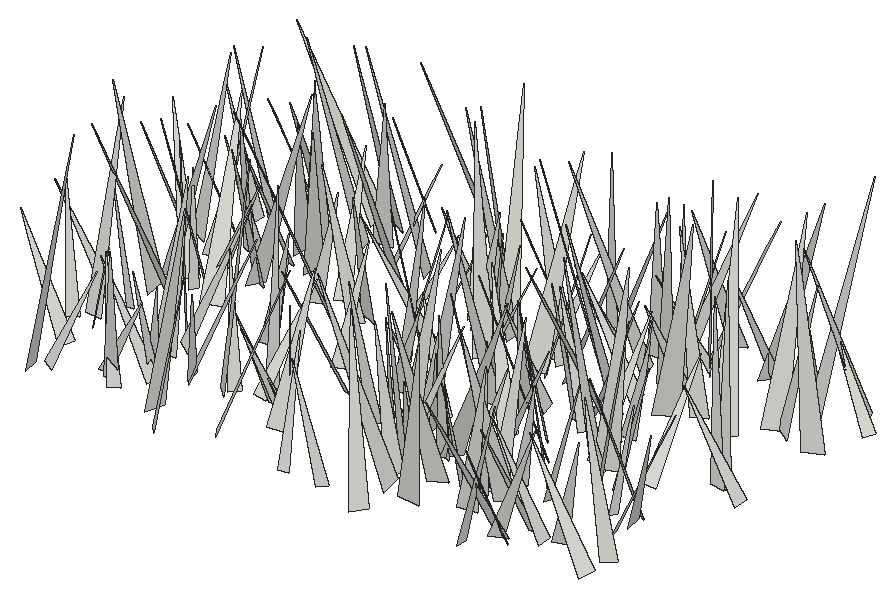
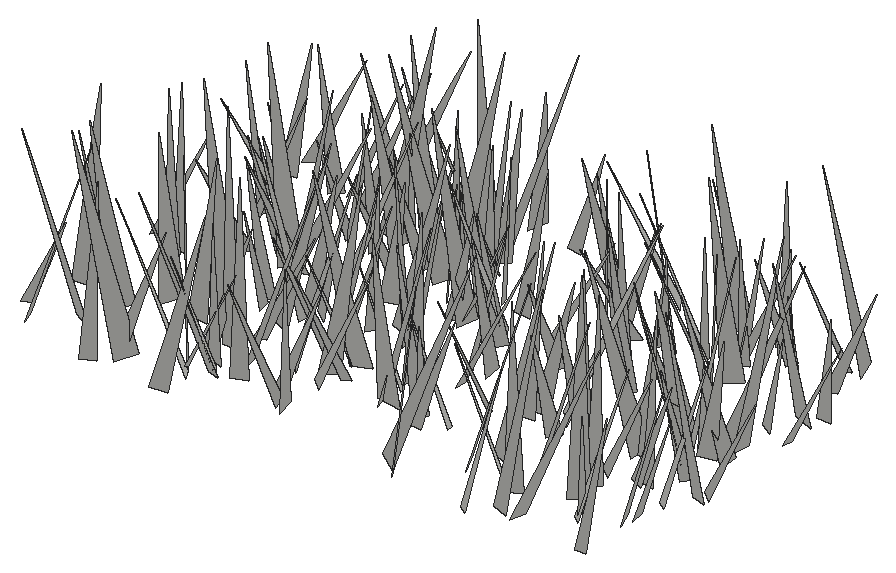
# SketchUp Ruby script. Lengths in inches.
U = 1.inch
M = Sketchup.active_model
def pt(a) = Geom::Point3d.new(a.map { |v| v * U })
def face(e, loops, mat)
  f = e.add_face(loops[0].map { |a| pt(a) })
  loops[1..].each { |l| e.add_face(l.map { |a| pt(a) }).erase! }
  f.material = f.back_material = mat if mat
  f
end
# faces: each face lists its corners as indices into pts; further lists are holes
def faces(e, pts, list, mat = nil) = list.each { |f| face(e, (f[0].is_a?(Array) ? f : [f]).map { |l| l.map { |i| pts[i] } }, mat) }
# xy, xz, yz: faces in a plane at the given z, y or x. An outline is a flat list of corners, or four numbers for a rectangle; further outlines are holes
def ring(l) = l.size == 4 ? [[l[0], l[1]], [l[2], l[1]], [l[2], l[3]], [l[0], l[3]]] : l.each_slice(2).to_a
def flat(e, list, mat, &to3) = list.each { |f| face(e, (f[0].is_a?(Array) ? f : [f]).map { |l| ring(l).map { |u, v| to3.(u, v) } }, mat) }
def xy(e, z, list, mat = nil) = flat(e, list, mat) { |x, y| [x, y, z] }
def xz(e, y, list, mat = nil) = flat(e, list, mat) { |x, z| [x, y, z] }
def yz(e, x, list, mat = nil) = flat(e, list, mat) { |y, z| [x, y, z] }
def lines(e, pts, list) = list.each { |a, b| e.add_line(pt(pts[a]), pt(pts[b])) }
# prism: a flat outline (further loops are holes) pulled along v
def prism(e, loops, v, mat = nil)
  f = face(e, loops, mat); d = Geom::Vector3d.new(v.map { |x| x * U })
  f.pushpull(f.normal.samedirection?(d) ? d.length : -d.length)
end
def box(e, o, s, mat = nil) = prism(e, [[o, [o[0] + s[0], o[1], o[2]], [o[0] + s[0], o[1] + s[1], o[2]], [o[0], o[1] + s[1], o[2]]]], [0, 0, s[2]], mat)
def at(x, y, z, deg = 0) = Geom::Transformation.translation(pt([x, y, z])) * Geom::Transformation.rotation(ORIGIN, Z_AXIS, deg.degrees)
def axes(o, x, y, z) = Geom::Transformation.new([*x, 0, *y, 0, *z, 0, *pt(o).to_a, 1])
def part(name) = M.definitions.add(name)
# library, detail: a bought-in or finely detailed component or shape, given as its bounding box
def library(name, o, s) = part(name).tap { |d| box(d.entities, o, s) }
def detail(e, o, s) = box(e.add_group.entities, o, s)
def put(e, d, t, mat = nil) = e.add_instance(d, t).tap { |i| i.material = mat if mat }
def group(e, t, mat = nil) = e.add_group.tap { |g| g.transformation = t; g.material = mat if mat }.entities
root = M.entities
c1 = part("fur_instance\#9")
p = [[0.8125,0,1.79],[0.67,-0.02,1.48],[0,-0.11,0],[0,0.11,0]]
faces(c1.entities,p,[[0,1,2,3]])
put(root,c1,axes([494.67,199.78,-21.66],[-2.5051,-3.46967,0.23869],[-3.39401,2.50314,0.76559],[0.75915,-0.25846,4.21047]))
put(root,c1,axes([494.2,200.04,-21.66],[-1.56968,-5.60909,0.11931],[-5.50885,1.51747,-1.1357],[-1.06238,0.41882,5.71278]))
put(root,c1,axes([481.14,198.01,-21.66],[-1.35537,3.98703,1.26023],[4.07237,0.95801,1.34893],[-0.94888,-1.58348,3.98921]))
put(root,c1,axes([468.15,197.01,-21.66],[3.87453,3.49507,1.24049],[3.40824,-4.0629,0.80191],[-1.46226,-0.20898,5.15601]))
put(root,c1,axes([484.87,197.01,-21.66],[-6.05277,2.56522,0.71834],[2.46544,6.06973,-0.90131],[1.00895,0.55714,6.51184]))
put(root,c1,axes([492.67,197.71,-21.66],[4.75143,0.92242,1.33841],[0.70934,-4.89704,0.85681],[-1.46255,0.62163,4.7637]))
put(root,c1,axes([486.59,199.97,-21.66],[1.17018,-6.95871,1.51726],[-7.0392,-0.89595,1.31981],[1.08411,1.69372,6.93189]))
put(root,c1,axes([462.06,200.32,-21.66],[-0.22733,-5.68785,1.31588],[-5.73337,0.46581,1.02292],[1.10075,1.2515,5.59972]))
put(root,c1,axes([501.49,199.53,-21.66],[-4.58774,2.19144,0.09862],[2.15217,4.45217,1.18567],[-0.42461,-1.11142,4.94408]))
put(root,c1,axes([477.98,197.96,-21.66],[0.35019,4.61175,0.40741],[4.56098,-0.41379,0.76359],[-0.79477,-0.34263,4.56155]))
put(root,c1,axes([493.86,199.77,-21.66],[3.98681,-3.04122,0.56389],[-3.08769,-3.85909,1.01744],[0.18196,1.14894,4.91004]))
put(root,c1,axes([484.51,200.73,-21.66],[-7.8071,-1.03462,1.04066],[-0.93299,7.84786,0.80297],[1.13267,-0.66693,7.83431]))
put(root,c1,axes([466.49,199.24,-21.66],[7.07212,-1.1156,2.41076],[-1.38462,-7.39913,0.63784],[-2.26697,1.03896,7.1311]))
put(root,c1,axes([457.67,199.39,-21.66],[1.33461,3.80482,0.72121],[3.71713,-1.04467,-1.36733],[1.08616,-1.09999,3.79319]))
put(root,c1,axes([456.9,198.5625,-21.66],[7.33246,2.99097,2.42144],[2.72494,-7.71469,1.27771],[-2.71735,0.33456,7.81527]))
put(root,c1,axes([496.68,201.2,-21.66],[-4.54566,0.43172,0.55069],[0.54174,4.46219,0.97364],[0.44289,-1.02717,4.4611]))
put(root,c1,axes([495.29,201.81,-21.66],[-1.01525,-4.25558,0.24661],[-4.20456,0.95799,-0.77812],[-0.70176,0.41691,4.30525]))
put(root,c1,axes([462.74,199.7,-21.66],[-1.18349,4.29439,0.91251],[4.36217,1.04349,0.74676],[-0.49586,-1.06979,4.39144]))
put(root,c1,axes([490.27,201.32,-21.66],[2.54415,-5.74451,1.38415],[-5.89364,-2.3587,1.04378],[0.42454,1.68081,6.19537]))
put(root,c1,axes([461.02,200.97,-21.66],[2.09245,-2.98815,0.44058],[-2.87886,-1.81085,1.39087],[0.91397,1.13723,3.37237]))
put(root,c1,axes([497.64,201.65,-21.66],[2.67886,-4.09104,0.57639],[-4.11516,-2.58128,0.80469],[0.36641,0.91951,4.82342]))
put(root,c1,axes([471.55,199.15,-21.66],[5.03516,3.5658,0.22039],[3.50469,-5.00395,0.89105],[-0.69327,0.6016,6.10523]))
put(root,c1,axes([486.55,203.04,-21.66],[1.44091,-6.85532,1.40735],[-6.89305,-1.6385,-0.92385],[-1.20912,1.1714,6.94393]))
put(root,c1,axes([464.1,202.01,-21.66],[-4.45422,0.97791,0.2811],[1.01486,4.3608,0.91044],[0.07343,-0.95002,4.4685]))
put(root,c1,axes([483.74,202.0625,-21.66],[3.52477,-3.78027,2.43443],[-3.94318,-4.08529,-0.63451],[-2.1606,1.28874,5.1295]))
put(root,c1,axes([463.72,202.64,-21.66],[-3.9744,-0.24759,1.6573],[0.13335,4.20562,0.94807],[1.67038,-0.92483,3.8676]))
put(root,c1,axes([491.44,203.78,-21.66],[2.47706,-6.70826,1.39737],[-6.69174,-2.68793,-1.04158],[-1.47445,0.92925,7.07472]))
put(root,c1,axes([463.31,203.02,-21.66],[0.57309,-4.07864,0.58369],[-4.03575,-0.43699,0.90892],[0.82985,0.69149,4.01716]))
put(root,c1,axes([501.54,201.7,-21.66],[-2.10663,5.00928,1.58804],[5.23429,1.84857,1.1125],[-0.46582,-1.88217,5.31913]))
put(root,c1,axes([456.88,202.27,-21.66],[-3.88022,2.75048,0.41463],[2.75578,3.70465,1.21426],[-0.37781,-1.22622,4.59857]))
put(root,c1,axes([483.27,204.12,-21.66],[4.01305,-1.4697,0.35123],[-1.33059,-3.90931,-1.15533],[-0.71618,-0.97223,4.11458]))
put(root,c1,axes([484.54,202.18,-21.66],[-3.5063,-5.04513,2.56803],[-5.65565,3.25438,-1.32851],[0.24851,2.88062,5.99854]))
put(root,c1,axes([474.17,203.42,-21.66],[-3.42009,-2.62307,1.97794],[-2.56254,3.91671,0.76324],[2.05575,0.51835,4.24205]))
put(root,c1,axes([465.8,203.89,-21.66],[3.91592,-0.46866,0.80636],[-0.26131,-3.89224,-0.99321],[-0.89531,-0.91384,3.81675]))
put(root,c1,axes([474.28,201.85,-21.66],[-2.07384,5.25709,1.74566],[5.26815,2.4479,-1.11335],[1.712,-1.16445,5.54061]))
put(root,c1,axes([488.96,202.72,-21.66],[0.98464,3.25356,1.70885],[3.23357,-1.6077,1.19779],[-1.74639,-1.14237,3.18127]))
put(root,c1,axes([472.22,204.58,-21.66],[-3.37943,-0.96857,0.84627],[-0.6019,3.29348,1.36586],[1.13667,-1.13567,3.23931]))
put(root,c1,axes([471.98,204.55,-21.66],[0.37183,-3.94608,0.38846],[-3.8933,-0.43727,-0.71534],[-0.75144,0.31297,3.89847]))
put(root,c1,axes([483.19,203.37,-21.66],[2.79379,4.96818,0.70977],[4.95175,-2.59669,-1.31495],[0.8165,-1.25148,5.54607]))
put(root,c1,axes([465.8,203.64,-21.66],[4.98455,3.49636,0.32674],[3.50629,-4.92427,-0.79656],[0.19289,-0.83908,6.03621]))
put(root,c1,axes([456.49,205.47,-21.66],[3.46775,1.51161,0.84573],[1.722,-3.21287,-1.3182],[-0.18693,-1.55498,3.54578]))
put(root,c1,axes([489.76,203.69,-21.66],[1.9045,4.44389,1.45881],[4.34306,-2.26488,1.22946],[-1.73613,-0.79091,4.67587]))
put(root,c1,axes([462.55,205.04,-21.66],[2.84119,-6.18581,2.36185],[-6.62137,-2.65127,1.02137],[0.00779,2.57322,6.73004]))
put(root,c1,axes([484.66,205.87,-21.66],[-1.17903,-5.46423,1.73554],[-5.62366,1.44698,0.7353],[1.11548,1.51937,5.54141]))
put(root,c1,axes([468.48,203.64,-21.66],[5.2038,5.70361,2.35891],[5.67233,-5.63566,1.11317],[-2.43315,-0.93989,7.64013]))
put(root,c1,axes([480.47,206.04,-21.66],[4.23333,1.58778,2.03705],[2.11026,-4.38143,-0.97034],[-1.48911,-1.69519,4.41595]))
put(root,c1,axes([499.62,206.57,-21.66],[4.97063,-0.22915,0.23226],[-0.15729,-4.7897,-1.3593],[-0.28585,-1.34904,4.78665]))
put(root,c1,axes([490.78,206.12,-21.66],[2.11868,-4.0714,0.72457],[-4.11944,-2.00647,0.77101],[0.3627,0.99394,4.52445]))
put(root,c1,axes([469.07,204.14,-21.66],[-4.35702,1.54483,0.37411],[1.45493,4.3157,-0.87633],[0.64002,0.7059,4.53896]))
put(root,c1,axes([485.13,206.16,-21.66],[6.73019,-3.63445,0.24466],[-3.63894,-6.68481,0.79754],[0.16506,0.81773,7.60715]))
put(root,c1,axes([490.28,204.5,-21.66],[-4.55508,3.55475,2.05706],[3.40532,4.98624,-1.07596],[2.29598,-0.34303,5.67691]))
put(root,c1,axes([478.51,206.57,-21.66],[-0.10037,-5.00985,1.67679],[-5.24561,-0.10471,-0.62683],[-0.62754,1.67652,4.9715]))
put(root,c1,axes([493.1,206.13,-21.66],[-3.89447,-3.70378,1.65585],[-4.00703,3.87088,-0.766],[0.63525,1.71028,5.3196]))
put(root,c1,axes([454.92,205.32,-21.66],[-0.91318,4.58049,0.90258],[4.61205,0.74242,0.89849],[-0.72428,-1.04754,4.5834]))
put(root,c1,axes([487.09,205.95,-21.66],[3.48145,-1.92251,0.90917],[-2.10367,-3.36896,0.93158],[-0.31179,1.26381,3.86636]))
put(root,c1,axes([499.5,204.74,-21.66],[4.18382,1.92252,0.07247],[1.86113,-4.08842,1.01327],[-0.48737,0.89131,4.49152]))
put(root,c1,axes([470.79,204.54,-21.66],[-0.63847,4.33122,0.11328],[4.14955,0.64421,-1.24344],[1.2464,0.07394,4.19773]))
put(root,c1,axes([493.51,205.45,-21.66],[3.85077,0.95797,1.10657],[0.6489,-3.90916,1.12606],[-1.31192,0.87829,3.80501]))
put(root,c1,axes([499.59,207.52,-21.66],[-3.22494,-3.97651,0.65226],[-4.0077,3.07801,-1.05003],[-0.42001,1.16258,5.01102]))
put(root,c1,axes([482.12,208.02,-21.66],[3.64013,-0.49009,0.65042],[-0.33955,-3.62113,-0.82821],[-0.74023,-0.74902,3.57838]))
put(root,c1,axes([483.43,208.125,-21.66],[-2.68709,-2.60275,1.28992],[-2.48203,2.97011,0.82256],[1.50922,0.25052,3.6494]))
put(root,c1,axes([470.54,206.14,-21.66],[1.55743,6.34801,1.89562],[6.44853,-1.89902,1.06134],[-1.51893,-1.55328,6.44953]))
put(root,c1,axes([497.95,206.67,-21.66],[-3.37958,0.77927,1.41196],[0.41341,3.58754,-0.99047],[1.55884,0.73803,3.32382]))
put(root,c1,axes([474.71,208.51,-21.66],[-2.69174,-3.80387,0.07847],[-3.66679,2.56798,-1.29661],[-1.01502,0.8106,4.47591]))
put(root,c1,axes([463.03,206.56,-21.66],[3.15484,4.86518,0.39731],[4.85003,-3.07066,-0.91053],[0.55227,-0.82578,5.72659]))
put(root,c1,axes([480.21,208.17,-21.66],[0.14436,6.2225,2.72909],[6.68972,0.34776,-1.14678],[1.18962,-2.71069,6.11762]))
put(root,c1,axes([455.85,206.25,-21.66],[1.84085,7.01016,1.12106],[6.97031,-2.00445,1.08846],[-1.34679,-0.79226,7.16563]))
put(root,c1,axes([480.9,209.3,-21.66],[-3.67924,-0.76157,0.35539],[-0.68587,3.64327,0.70657],[0.48566,-0.62424,3.6902]))
put(root,c1,axes([454.88,209.08,-21.66],[-4.32306,0.06447,0.02072],[0.06687,4.27292,0.65655],[0.01068,-0.65679,4.2734]))
put(root,c1,axes([457.12,208.43,-21.66],[0.68239,3.8164,1.4602],[3.78451,-1.14857,1.23331],[-1.54098,-1.13076,3.67553]))
put(root,c1,axes([490.18,209.66,-21.66],[-4.77204,-4.71706,0.72174],[-4.75307,4.60775,-1.31181],[-0.42413,1.43592,6.58044]))
put(root,c1,axes([487.72,208.02,-21.66],[4.13014,0.16234,0.60229],[0.00137,-4.03539,1.07832],[-0.62379,1.06603,3.99019]))
put(root,c1,axes([461.8125,208.27,-21.66],[3.98122,4.30027,2.75674],[4.211,-4.74141,1.31475],[-2.89126,-0.98426,5.71085]))
put(root,c1,axes([466.98,210.17,-21.66],[2.1882,-4.93746,0.79161],[-4.93819,-1.99768,1.19031],[0.78701,1.19336,5.26781]))
put(root,c1,axes([457.93,211.48,-21.66],[-3.16334,-6.14078,0.476],[-6.132,3.08971,-0.89149],[-0.57823,0.82883,6.8499]))
put(root,c1,axes([477.02,210.57,-21.66],[2.31724,-3.70248,0.25487],[-3.62607,-2.19471,1.08527],[0.79054,0.78602,4.23086]))
put(root,c1,axes([480.6,209.57,-21.66],[7.15421,-1.9799,2.12173],[-2.22149,-7.36827,0.61487],[-1.86728,1.18029,7.39761]))
put(root,c1,axes([495.05,208.78,-21.66],[4.98467,2.72403,1.68688],[2.57744,-5.26236,0.88159],[-1.90334,0.00786,5.61161]))
put(root,c1,axes([481.6,209.87,-21.66],[1.42744,-3.53628,2.17287],[-3.81125,-2.02664,-0.79456],[-1.64348,1.62839,3.72982]))
put(root,c1,axes([495.93,209.5,-21.66],[4.26152,0.65659,1.09682],[0.47447,-4.35714,0.76482],[-1.18701,0.6156,4.24343]))
put(root,c1,axes([466.57,211.03,-21.66],[1.64053,-3.56149,0.70323],[-3.59089,-1.47867,0.88831],[0.53314,0.99969,3.81922]))
put(root,c1,axes([494.1,209.99,-21.66],[-7.25051,-1.24633,1.39987],[-1.43303,7.2913,-0.93068],[1.20805,1.16894,7.29774]))
put(root,c1,axes([456.72,211.52,-21.66],[6.73753,-0.02978,4.19134],[0.53715,-7.86314,-0.91932],[-4.15689,-1.06433,6.67458]))
put(root,c1,axes([482.75,211.85,-21.66],[-2.78076,-3.999,1.01738],[-3.97731,2.92434,0.62365],[1.09912,0.46468,4.83071]))
put(root,c1,axes([493.87,210.94,-21.66],[-3.12669,6.25889,3.83958],[6.87271,3.96367,-0.86451],[2.58493,-2.9678,6.9428]))
put(root,c1,axes([477.66,209.22,-21.66],[5.27233,3.79468,0.9806],[3.62511,-5.34626,1.19781],[-1.48988,0.42019,6.38454]))
put(root,c1,axes([486.17,210.6,-21.66],[-2.8304,4.89567,0.80261],[4.94903,2.72215,0.8485],[-0.34477,-1.11592,5.59096]))
put(root,c1,axes([488.59,211.5625,-21.66],[-3.38469,-3.26483,1.22467],[-3.48648,3.19729,-1.11215],[0.05857,1.65326,4.56929]))
put(root,c1,axes([503.34,212.88,-21.66],[-4.40105,0.97982,0.44244],[1.06612,4.21791,1.26401],[0.13855,-1.33202,4.328]))
put(root,c1,axes([459.09,213.71,-21.66],[-4.71687,-4.84842,1.35584],[-4.8132,4.8877,0.73342],[1.47602,0.44449,6.72444]))
put(root,c1,axes([483.24,213.02,-21.66],[-1.73003,-6.76572,2.01517],[-7.01807,1.42401,-1.24409],[-0.76325,2.2419,6.8717]))
put(root,c1,axes([472.29,210.64,-21.66],[-3.28423,2.60896,0.74342],[2.31234,3.30268,-1.37511],[1.4186,0.65664,3.96257]))
put(root,c1,axes([491.95,214.48,-21.66],[-3.14306,-6.22127,0.26286],[-6.12359,3.03481,-1.39417],[-1.12913,0.859,6.8293]))
put(root,c1,axes([484.73,214.18,-21.66],[4.79188,-1.27621,1.00499],[-1.01396,-4.79557,-1.25507],[-1.26909,-0.98723,4.79746]))
put(root,c1,axes([497.36,210.99,-21.66],[-1.55041,4.4226,0.08121],[4.26043,1.51619,-1.23272],[1.18941,0.33394,4.52145]))
put(root,c1,axes([492.85,211.15,-21.66],[-0.26942,5.43204,0.24352],[5.36362,0.30555,-0.88154],[0.89325,-0.19629,5.36679]))
put(root,c1,axes([459.84,213.29,-21.66],[4.56637,-2.19972,0.30987],[-2.21681,-4.46657,0.96025],[0.14341,0.99877,4.97679]))
put(root,c1,axes([486.03,214.8125,-21.66],[-4.24869,-0.73201,1.00331],[-0.4187,4.21079,1.29914],[1.16925,-1.15205,4.11089]))
put(root,c1,axes([481.91,214.1,-21.66],[6.17707,1.48648,1.9777],[1.80034,-6.34915,-0.85095],[-1.69697,-1.32504,6.29616]))
put(root,c1,axes([458.74,212.88,-21.66],[-3.88558,0.60859,0.85055],[0.43871,3.91906,-0.80001],[0.9494,0.67978,3.85072]))
put(root,c1,axes([467.9375,215.39,-21.66],[-5.60021,-5.8066,0.30959],[-5.79691,5.54128,-0.92996],[-0.45638,0.8674,8.01337]))
put(root,c1,axes([489.79,214.09,-21.66],[-3.61147,3.35043,1.62323],[3.67501,3.56996,0.80783],[0.59541,-1.71259,4.85958]))
put(root,c1,axes([476.78,213.96,-21.66],[-4.01127,-3.66818,1.32519],[-3.89401,3.87381,-1.06408],[0.2199,1.68524,5.33044]))
put(root,c1,axes([500.87,213.57,-21.66],[1.52535,6.05061,2.3847],[6.37233,-1.8801,0.69429],[-1.30004,-2.1163,6.20117]))
put(root,c1,axes([456.25,213.4375,-21.66],[6.19902,-0.22924,1.58295],[-0.50577,-6.29178,1.06951],[-1.51739,1.16065,6.11037]))
put(root,c1,axes([460.92,212,-21.66],[-3.48559,6.14429,0.41822],[6.11379,3.5101,-0.61419],[0.74073,-0.05879,7.03735]))
put(root,c1,axes([461.41,216.17,-21.66],[-1.87294,-5.65903,1.00828],[-5.62978,2.02003,0.87988],[1.16052,0.66634,5.89562]))
put(root,c1,axes([492.45,215.08,-21.66],[1.94389,-4.04886,0.80465],[-4.08173,-1.75236,1.04312],[0.61659,1.16421,4.36851]))
put(root,c1,axes([475.91,216.14,-21.66],[-5.4104,-1.19331,0.05848],[-1.15989,5.3113,1.06983],[0.28647,-1.03242,5.43616]))
put(root,c1,axes([475.28,213.67,-21.66],[5.18015,0.30458,2.40247],[-0.20645,-5.59667,1.15468],[-2.41288,1.13276,5.059]))
put(root,c1,axes([489.07,215.66,-21.66],[6.07626,0.90493,0.17774],[0.92213,-5.94508,-1.25588],[0.01299,-1.26833,6.01354]))
put(root,c1,axes([488.4375,214.73,-21.66],[-2.6227,-3.62693,1.52989],[-3.9333,2.34177,-1.19122],[-0.15598,1.93268,4.31442]))
put(root,c1,axes([501.28,213.7,-21.66],[1.52535,6.57132,1.88983],[6.63248,-1.89273,1.22809],[-1.66251,-1.52175,6.63331]))
put(root,c1,axes([457.66,213.78,-21.66],[-2.82943,5.24506,0.49337],[5.22615,2.72388,1.01368],[-0.66438,-0.91081,5.87271]))
put(root,c1,axes([469.74,216.86,-21.66],[-1.23587,-5.65616,0.92472],[-5.5483,1.41785,1.25724],[1.43652,0.61007,5.65145]))
put(root,c1,axes([469.59,215.88,-21.66],[0.51311,-4.91857,2.52241],[-5.22585,-1.25725,-1.38854],[-1.80151,2.24614,4.74633]))
put(root,c1,axes([489.62,217.34,-21.66],[-2.51805,-6.35566,1.6356],[-6.55451,2.34778,-0.96776],[-0.32873,1.87181,6.76746]))
put(root,c1,axes([465.88,216.34,-21.66],[2.99214,-2.75371,1.44433],[-3.06357,-2.95389,0.71483],[-0.53251,1.52102,4.0031]))
put(root,c1,axes([461.41,215.83,-21.66],[7.18053,-1.42617,1.70446],[-1.71997,-7.21687,1.20732],[-1.40743,1.54336,7.22055]))
put(root,c1,axes([492.05,215.99,-21.66],[3.63401,0.67625,1.41653],[0.37628,-3.84346,0.86953],[-1.5239,0.6636,3.59267]))
put(root,c1,axes([456.85,216.88,-21.66],[2.18192,-3.03993,1.35648],[-3.32882,-1.9865,0.90262],[0.01238,1.6293,3.63142]))
put(root,c1,axes([454.59,217.7,-21.66],[-2.53868,-3.44184,0.53172],[-3.38696,2.28677,-1.36858],[-0.81085,1.22404,4.05193]))
put(root,c1,axes([457.81,215.94,-21.66],[5.71474,5.0925,1.62445],[5.00095,-5.93344,1.00766],[-1.88756,-0.30227,7.58791]))
put(root,c1,axes([458.46,218.88,-21.66],[-1.39495,-5.41554,1.57218],[-5.52882,1.63221,0.71678],[1.10996,1.3242,5.54619]))
put(root,c1,axes([463.23,219.47,-21.66],[5.78336,-2.78291,1.02515],[-2.6557,-5.85961,-0.92463],[-1.32013,-0.40388,6.35113]))
put(root,c1,axes([492.52,218.78,-21.66],[5.49312,-5.94068,1.74056],[-6.16398,-5.4638,0.80479],[-0.57141,1.8305,8.05098]))
put(root,c1,axes([472.39,217.61,-21.66],[2.24479,3.42751,0.35228],[3.3467,-2.06895,-1.19586],[0.81948,-0.93948,3.91878]))
put(root,c1,axes([456.08,220.36,-21.66],[-3.01664,-4.03882,0.35129],[-3.9528,3.02747,0.86334],[0.90049,-0.2406,4.96657]))
put(root,c1,axes([478.4,218.99,-21.66],[3.77978,1.93812,0.15141],[1.88384,-3.56988,-1.33157],[0.48001,-1.25124,4.0336]))
put(root,c1,axes([461.59,219.26,-21.66],[-2.18116,-3.44946,0.52539],[-3.41914,1.9894,-1.13316],[-0.6959,1.0372,3.92074]))
put(root,c1,axes([454.67,218.44,-21.66],[2.76981,6.05425,2.08045],[6.39697,-2.70498,-0.64491],[-0.24704,-2.16406,6.62646]))
put(root,c1,axes([459.19,219.125,-21.66],[-0.15517,3.72025,1.9318],[3.94772,-0.52047,1.31942],[-1.40985,-1.86683,3.48188]))
put(root,c1,axes([489.59,219.44,-21.66],[-4.14397,2.00475,0.46664],[2.04964,3.92263,1.34951],[-0.1891,-1.41534,4.40117]))
put(root,c1,axes([478.7,217.54,-21.66],[-7.32985,2.37013,1.25415],[2.21242,7.40801,-1.06942],[1.51512,0.64882,7.62892]))
put(root,c1,axes([476.6,219.59,-21.66],[0.64184,-5.02818,1.67754],[-5.1921,-0.25617,1.21871],[1.0672,1.77778,4.9203]))
put(root,c1,axes([461.03,221.11,-21.66],[5.82388,-2.11588,0.96568],[-1.89422,-5.82584,-1.34106],[-1.34958,-0.95373,6.04946]))
put(root,c1,axes([467.08,217.61,-21.66],[-3.56448,3.67904,0.44666],[3.56023,3.5714,-1.00507],[1.02934,0.38746,5.02301]))
put(root,c1,axes([467.98,222.01,-21.66],[-2.86218,-6.85746,0.77217],[-6.83354,2.93291,0.71683],[0.96112,0.43167,7.39614]))
put(root,c1,axes([482.29,218.25,-21.66],[-1.03239,7.59334,1.92082],[7.72051,1.31303,-1.04105],[1.31985,-1.74108,7.59215]))
put(root,c1,axes([483.31,220.25,-21.66],[-5.98098,3.27291,2.42019],[3.72115,6.13978,0.89298],[1.64993,-1.98304,6.75918]))
put(root,c1,axes([484.82,218.29,-21.66],[4.77629,1.47467,0.59608],[1.29577,-4.70156,1.24867],[-0.92247,1.03128,4.84029]))
put(root,c1,axes([483.25,218.02,-21.66],[3.76197,3.17485,0.58422],[2.97684,-3.75885,1.25811],[-1.24876,0.60394,4.75913]))
put(root,c1,axes([485.8,220.67,-21.66],[-5.67662,-5.13617,1.32256],[-5.29359,5.60645,-0.94818],[0.32758,1.59402,7.59639]))
put(root,c1,axes([490.38,221.4,-21.66],[-1.23371,-7.71978,2.49826],[-7.92295,1.69122,1.31342],[1.75022,2.21429,7.70662]))
put(root,c1,axes([494.3125,219.95,-21.66],[-1.23354,6.12021,2.2306],[6.48252,0.93032,1.03231],[-0.63996,-2.37312,6.15735]))
put(root,c1,axes([491.61,221.95,-21.66],[1.92833,-3.54748,0.58332],[-3.33012,-2.01195,-1.22706],[-1.35468,-0.10385,3.84674]))
put(root,c1,axes([477.5,220.78,-21.66],[2.1321,2.91958,1.28602],[3.18698,-1.87905,-1.01782],[0.14466,-1.63367,3.46899]))
put(root,c1,axes([472.9375,220.93,-21.66],[3.88446,1.51086,0.00017],[1.46105,-3.75628,-1.06181],[0.38475,-0.98965,4.03042]))
put(root,c1,axes([502.85,220.85,-21.66],[1.15068,-6.84996,3.27998],[-7.48842,-1.57649,-0.66528],[-1.26644,3.09791,6.914]))
put(root,c1,axes([488.1,222.46,-21.66],[-7.76303,-2.55675,1.09489],[-2.43873,7.81802,0.96517],[1.33728,-0.58482,8.11604]))
put(root,c1,axes([483.13,221.73,-21.66],[-3.10953,-4.00727,0.37973],[-3.98696,3.00024,-0.98706],[-0.55366,0.90108,4.97525]))
put(root,c1,axes([460.71,223.05,-21.66],[2.24537,-6.9608,0.71668],[-6.96969,-2.1575,0.8813],[0.62434,0.94895,7.26069]))
put(root,c1,axes([497.1,219.08,-21.66],[5.53383,-2.65462,5.00816],[-4.23304,-6.59023,1.18414],[-3.76962,3.5034,6.0223]))
put(root,c1,axes([478.58,220.6,-21.66],[-7.60093,-1.69118,1.08047],[-1.85126,7.54274,-1.21718],[0.77483,1.43129,7.69108]))
put(root,c1,axes([481.97,220.15,-21.66],[0.26684,4.21608,0.5662],[4.07293,-0.08948,-1.25314],[1.22767,-0.6195,4.03438]))
put(root,c1,axes([474.83,222.17,-21.66],[0.84597,-3.78981,1.14812],[-3.67965,-1.18614,-1.20406],[-1.46323,0.79177,3.69169]))
put(root,c1,axes([499.85,221.57,-21.66],[3.01267,4.99828,1.819],[5.31773,-2.78497,-1.15474],[0.11548,-2.15148,5.72063]))
put(root,c1,axes([475.11,221,-21.66],[-3.68366,1.92684,0.76086],[1.83141,3.75443,-0.64122],[0.96827,0.22919,4.10742]))
put(root,c1,axes([484.4,223.94,-21.66],[1.61464,-3.26071,0.69447],[-2.99454,-1.75765,-1.29032],[-1.46534,-0.00102,3.40211]))
put(root,c1,axes([456.35,222.56,-21.66],[-4.63616,-0.58897,0.33378],[-0.62989,4.59941,-0.63319],[0.24806,0.67142,4.63033]))
put(root,c1,axes([499.08,221.63,-21.66],[-4.71435,5.59524,2.23508],[5.56124,5.13291,-1.11952],[2.31839,-0.93486,7.23039]))
put(root,c1,axes([487.35,224.36,-21.66],[0.93072,-6.54849,1.55591],[-6.7031,-0.75944,0.81335],[0.60996,1.64631,6.5641]))
put(root,c1,axes([477.91,220.91,-21.66],[-0.32528,8.12923,0.88129],[8.06717,0.17507,1.36272],[-1.33486,-0.92294,8.0208]))
put(root,c1,axes([459.21,225.21,-21.66],[-3.58338,-3.97137,0.418],[-3.89573,3.60001,0.80641],[0.87736,-0.23507,5.28792]))
put(root,c1,axes([464.53,224.91,-21.66],[2.07468,-5.92746,1.15005],[-6.03286,-1.98482,0.6533],[0.24901,1.299,6.24598]))
put(root,c1,axes([466.5,223.61,-21.66],[3.8277,2.64651,0.3376],[2.6435,-3.68235,-1.10521],[0.36045,-1.09797,4.52038]))
put(root,c1,axes([456.77,223.35,-21.66],[-5.59376,-1.56322,0.76508],[-1.67452,5.53596,-0.93185],[0.47433,1.10847,5.73284]))
put(root,c1,axes([469.09,223.72,-21.66],[-7.24522,-3.15461,1.03201],[-3.28219,7.17812,-1.10079],[0.49381,1.42581,7.82516]))
put(root,c1,axes([463.77,224,-21.66],[-6.93543,-2.32629,0.88421],[-2.41004,6.93097,-0.66862],[0.62063,0.91853,7.28456]))
put(root,c1,axes([490.93,225.42,-21.66],[-3.84083,-1.16764,0.10273],[-1.10793,3.73134,0.98769],[0.38264,-0.91633,3.89099]))
put(root,c1,axes([490,223.53,-21.66],[1.00537,5.49165,1.69021],[5.63183,-1.28199,0.81538],[-1.13911,-1.49133,5.52306]))
put(root,c1,axes([490.86,225.27,-21.66],[5.50119,4.10651,2.99111],[4.73487,-5.74232,-0.82461],[-1.84151,-2.49711,6.81516]))
put(root,c1,axes([504.24,224.9,-21.66],[-3.16167,2.60611,0.16715],[2.5519,3.02748,1.0668],[-0.55458,-0.92652,3.956]))
put(root,c1,axes([502.91,226.51,-21.66],[-6.09562,-2.74651,0.83103],[-2.67616,6.14538,0.68045],[1.03541,-0.28555,6.65108]))
put(root,c1,axes([473.25,226.84,-21.66],[-4.28269,-7.03673,0.88853],[-7.06243,4.13524,-1.29164],[-0.65353,1.42504,8.13564]))
put(root,c1,axes([495.52,226.59,-21.66],[-0.21744,-4.53269,0.61909],[-4.46943,0.07824,-0.99696],[-0.9761,0.65149,4.42703]))
put(root,c1,axes([463.72,227.35,-21.66],[-3.21608,-6.87634,1.40534],[-6.91778,3.36666,0.64196],[1.18463,0.99184,7.56406]))
put(root,c1,axes([459.44,224.33,-21.66],[-4.54245,-0.30979,1.16713],[-0.64985,4.4561,-1.34644],[1.01777,1.46262,4.34936]))
put(root,c1,axes([489.15,224.52,-21.66],[3.76049,3.04894,0.61025],[2.98388,-3.80785,0.6375],[-0.87456,0.11813,4.79905]))
put(root,c1,axes([489.02,224.95,-21.66],[3.55811,5.92159,0.8478],[5.93377,-3.36884,-1.37307],[0.75783,-1.4247,6.77052]))
put(root,c1,axes([482.8,225.375,-21.66],[-5.66532,-0.50223,1.85308],[-0.88322,5.80808,-1.12609],[1.70472,1.34012,5.57494]))
put(root,c1,axes([483.44,225.19,-21.66],[4.63443,1.21877,0.59299],[1.09033,-4.6073,0.94811],[-0.80513,0.77609,4.69728]))
put(root,c1,axes([494.73,226.66,-21.66],[7.07738,-3.29601,0.99897],[-3.4049,-7.03943,0.89669],[-0.51794,1.23844,7.75557]))
put(root,c1,axes([462.375,227.22,-21.66],[-7.38136,0.22251,0.33251],[0.26326,7.32737,0.9407],[0.30128,-0.95116,7.32455]))
put(root,c1,axes([456.39,228.28,-21.66],[-0.44013,-4.40012,0.04518],[-4.35564,0.44209,0.62427],[0.62566,-0.01764,4.37779]))
put(root,c1,axes([490.32,225.99,-21.66],[5.45999,3.37552,0.2587],[3.37248,-5.38033,-0.97518],[0.29572,-0.96459,6.34466]))
put(root,c1,axes([496.49,228.42,-21.66],[1.50872,-5.62418,0.24688],[-5.60162,-1.47433,0.64555],[0.56049,0.40439,5.78713]))
put(root,c1,axes([472.18,227.71,-21.66],[4.90048,2.76624,3.25214],[3.64641,-5.28694,-0.99757],[-2.22086,-2.5767,5.5382]))
put(root,c1,axes([490.55,228.66,-21.66],[1.73584,-5.70606,0.92261],[-5.63591,-1.88469,-1.0526],[-1.28332,0.55882,5.87063]))
put(root,c1,axes([465.66,228.71,-21.66],[-3.10311,-4.08719,0.56583],[-3.96021,3.14894,1.02739],[1.15846,-0.18348,5.02781]))
put(root,c1,axes([499.88,224.68,-21.66],[3.85814,7.37241,1.12129],[7.37277,-3.96052,0.67189],[-1.11889,-0.67587,8.29374]))
